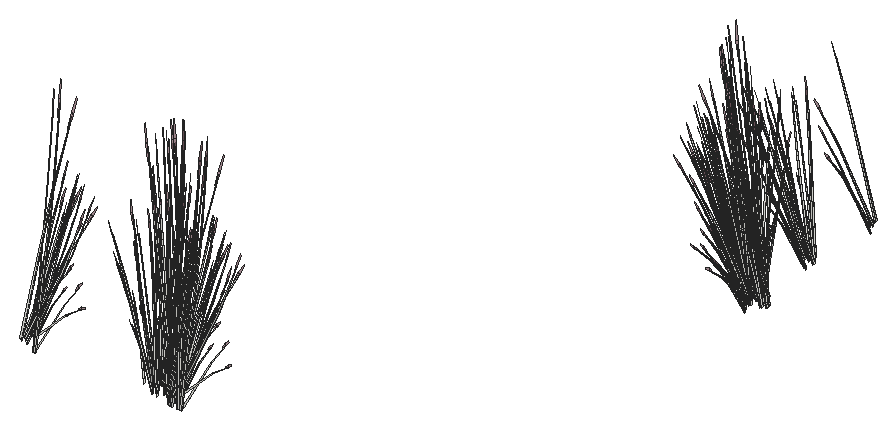
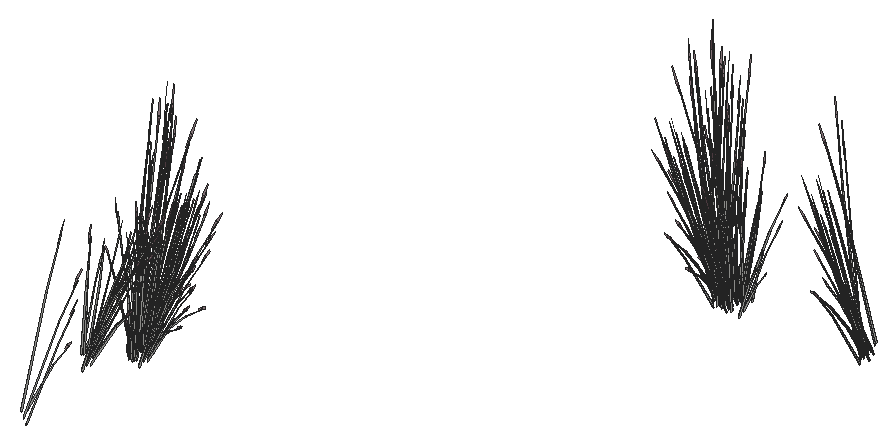
# SketchUp Ruby script. Lengths in inches.
U = 1.inch
M = Sketchup.active_model
def pt(a) = Geom::Point3d.new(a.map { |v| v * U })
def face(e, loops, mat)
  f = e.add_face(loops[0].map { |a| pt(a) })
  loops[1..].each { |l| e.add_face(l.map { |a| pt(a) }).erase! }
  f.material = f.back_material = mat if mat
  f
end
# faces: each face lists its corners as indices into pts; further lists are holes
def faces(e, pts, list, mat = nil) = list.each { |f| face(e, (f[0].is_a?(Array) ? f : [f]).map { |l| l.map { |i| pts[i] } }, mat) }
# xy, xz, yz: faces in a plane at the given z, y or x. An outline is a flat list of corners, or four numbers for a rectangle; further outlines are holes
def ring(l) = l.size == 4 ? [[l[0], l[1]], [l[2], l[1]], [l[2], l[3]], [l[0], l[3]]] : l.each_slice(2).to_a
def flat(e, list, mat, &to3) = list.each { |f| face(e, (f[0].is_a?(Array) ? f : [f]).map { |l| ring(l).map { |u, v| to3.(u, v) } }, mat) }
def xy(e, z, list, mat = nil) = flat(e, list, mat) { |x, y| [x, y, z] }
def xz(e, y, list, mat = nil) = flat(e, list, mat) { |x, z| [x, y, z] }
def yz(e, x, list, mat = nil) = flat(e, list, mat) { |y, z| [x, y, z] }
def lines(e, pts, list) = list.each { |a, b| e.add_line(pt(pts[a]), pt(pts[b])) }
# prism: a flat outline (further loops are holes) pulled along v
def prism(e, loops, v, mat = nil)
  f = face(e, loops, mat); d = Geom::Vector3d.new(v.map { |x| x * U })
  f.pushpull(f.normal.samedirection?(d) ? d.length : -d.length)
end
def box(e, o, s, mat = nil) = prism(e, [[o, [o[0] + s[0], o[1], o[2]], [o[0] + s[0], o[1] + s[1], o[2]], [o[0], o[1] + s[1], o[2]]]], [0, 0, s[2]], mat)
def at(x, y, z, deg = 0) = Geom::Transformation.translation(pt([x, y, z])) * Geom::Transformation.rotation(ORIGIN, Z_AXIS, deg.degrees)
def axes(o, x, y, z) = Geom::Transformation.new([*x, 0, *y, 0, *z, 0, *pt(o).to_a, 1])
def part(name) = M.definitions.add(name)
# library, detail: a bought-in or finely detailed component or shape, given as its bounding box
def library(name, o, s) = part(name).tap { |d| box(d.entities, o, s) }
def detail(e, o, s) = box(e.add_group.entities, o, s)
def put(e, d, t, mat = nil) = e.add_instance(d, t).tap { |i| i.material = mat if mat }
def group(e, t, mat = nil) = e.add_group.tap { |g| g.transformation = t; g.material = mat if mat }.entities
root = M.entities
M.materials.add("LightPink_Translucent").color = [144, 107, 117]
M.materials["LightPink_Translucent"].alpha = 0.75
c1 = part("blade")
p = [[2.15,0.21,22],[0,0.17,0],[0.09,0.45,0],[2.18,0.31,22],[2.29,0.31,22],[0.38,0.45,0],
  [2.48,0.24,33],[2.49,0.24,33],[2.48,0.22,33]]
faces(c1.entities,p,[[0,1,2,3],[4,5,2,3],[6,3,4,7],[8,0,3,6]])
c2 = part("seeds")
p = [[0.3,-0.1,1.38],[-0.01,-0.03,1.59],[-0.01,-0.03,0.03],[0.14,-0.07,-0.07],[0.29,-0.03,3],[0.15,0.01,3.11]]
faces(c2.entities,p,[[0,1,2,3],[1,0,4,5]],"LightPink_Translucent")
c3 = part("blade with seeds")
put(c3.entities,c1,at(0,0,0))
put(c3.entities,c2,axes([2.4,0.25,30.99],[1.5799,-0.05474,1.17369],[-0.12525,1.92788,0.29478],[-0.07173,-0.02425,1.56792]))
put(root,c3,axes([421.09,14.8,-3.8],[0.76598,0.27433,0],[-0.36864,0.57001,0],[0,0,1.74954]))
put(root,c3,axes([386.9,14.48,-1.28],[0.16299,-0.01033,1.74944],[0.44707,-0.47471,-0.27667],[0.28992,0.06266,0.14031]))
put(root,c3,axes([423.32,14.48,-1.28],[0.16299,-0.01033,1.74944],[0.44707,-0.47471,-0.27667],[0.28992,0.06266,0.14031]))
put(root,c3,axes([421.4,15.4,-3.81],[-0.46912,-0.61443,-0.05142],[0.79476,-0.34146,0.51607],[-0.19584,0.0585,1.6363]))
put(root,c3,axes([421.23,13.92,-3.38],[0.56134,0.36712,0.1448],[-0.46823,0.41419,-0.41347],[-0.13033,0.05599,1.26744]))
put(root,c3,axes([416.8,14.01,-1.27],[-0.18844,-0.56237,0.48003],[0.73919,-0.0976,0.3958],[-0.21785,0.13226,0.9933]))
put(root,c3,axes([416.65,13.9,-1.27],[-0.52161,-0.25698,0.0643],[0.30368,-0.36595,0.50621],[-0.16723,0.11831,0.77189]))
put(root,c3,axes([416.89,13.23,-2.125],[0.26363,-0.12925,1.71376],[0.22195,0.59723,0.13857],[-0.41388,0.13498,0.73262]))
put(root,c3,axes([386.27,14.55,-1.02],[0.75952,0.01471,-0.71045],[-0.05101,0.61953,0.08574],[0.32177,0.06538,1.00501]))
put(root,c3,axes([422.6875,14.55,-1.02],[0.75952,0.01471,-0.71045],[-0.05101,0.61953,0.08574],[0.32177,0.06538,1.00501]))
put(root,c3,axes([421.83,15.05,-3.52],[0.7111,-0.30552,0.49651],[0.42504,0.54784,0],[-0.16196,0.06958,1.57504]))
put(root,c3,axes([420.82,14.57,-3.71],[0.33034,0.70197,-0.06012],[-0.94388,0.24598,0],[0.01154,0.02451,1.72173]))
put(root,c3,axes([421.19,15.32,-3.97],[-0.70886,-0.15119,-0.30978],[0.17848,-0.53243,0.30978],[-0.1429,0.0614,1.38974]))
put(root,c3,axes([416.07,14.24,-3.41],[0.26405,0.05016,1.43002],[0.17019,0.51235,-0.30754],[-0.35868,0.0959,0.61141]))
put(root,c3,axes([417.25,13.83,-0.95],[0.66138,-0.08733,0.35414],[0.17464,0.49921,-0.4572],[-0.18953,0.13408,0.87481]))
put(root,c3,axes([387.51,13.29,-3.625],[0.95008,0,0],[0,0.68292,-0.51607],[0,0.15554,1.63711]))
put(root,c3,axes([423.93,13.29,-3.625],[0.95008,0,0],[0,0.68292,-0.51607],[0,0.15554,1.63711]))
put(root,c3,axes([414.71,13.6,-1.29],[0.09697,0.01639,1.77383],[0.29997,0.53988,-0.16761],[-0.1985,0.1417,0.31391]))
put(root,c3,axes([423.55,13.64,-3.8],[-0.94962,-0.00489,-0.04976],[0,-0.68292,0.49943],[-0.02984,0.15546,1.58352]))
put(root,c3,axes([421.49,13.05,-3.33],[0.85568,0.29155,-0.29095],[-0.41201,0.61537,-0.50002],[0.02689,0.15109,1.59708]))
put(root,c3,axes([415.52,15.32,-3.23],[0.31665,-0.27694,1.1486],[0.12495,0.43841,0.84392],[-0.22883,0.0785,0.25299]))
put(root,c3,axes([386.72,14.81,-1.47],[0.43232,0.38257,-0.35414],[-0.49364,0.36215,0.4572],[0.25081,0.0551,0.87481]))
put(root,c3,axes([423.14,14.81,-1.47],[0.43232,0.38257,-0.35414],[-0.49364,0.36215,0.4572],[0.25081,0.0551,0.87481]))
put(root,c3,axes([423.35,13.74,-3.97],[-0.53038,0.38124,-0.30978],[-0.53038,-0.38124,0.30978],[0,0.1228,1.38974]))
put(root,c3,axes([421.0625,13.78,-3.33],[0.08854,0.69723,-0.29095],[-0.92215,0.04216,-0.50002],[-0.16238,0.09287,1.59708]))
put(root,c3,axes([386.5,14.95,-1.27],[-0.03826,0.46465,0.0643],[-0.57772,-0.01274,0.50621],[0.2213,0.04862,0.77189]))
put(root,c3,axes([422.92,14.95,-1.27],[-0.03826,0.46465,0.0643],[-0.57772,-0.01274,0.50621],[0.2213,0.04862,0.77189]))
put(root,c3,axes([421.4,13.51,-3.79],[-0.36864,0.55059,-0.44739],[-0.76598,-0.26498,0.21531],[0,0.12692,1.43643]))
put(root,c3,axes([416.71,14.12,-1.47],[-0.66138,0.08733,-0.35414],[-0.17464,-0.49921,0.4572],[-0.18953,0.13408,0.87481]))
put(root,c3,axes([386.56,14.81,-1.27],[-0.56024,0.40262,0.48003],[-0.48318,-0.42758,0.3958],[0.26285,0.07427,0.9933]))
put(root,c3,axes([422.97,14.81,-1.27],[-0.56024,0.40262,0.48003],[-0.48318,-0.42758,0.3958],[0.26285,0.07427,0.9933]))
put(root,c3,axes([415.75,15.24,-0.35],[0.67048,0.16311,-0.06488],[-0.20625,0.50201,-0.29416],[-0.10966,0.07622,0.97024]))
put(root,c3,axes([420.51,14.3125,-3.94],[-0.51177,0.45928,-0.62353],[-0.63575,-0.41646,-0.16365],[-0.20507,0.11457,1.37633]))
put(root,c3,axes([384.77,15.27,-0.95],[-0.11735,-0.49217,0.35414],[0.67083,-0.12996,-0.4572],[0.18018,0.14104,0.87481]))
put(root,c3,axes([421.19,15.27,-0.95],[-0.11735,-0.49217,0.35414],[0.67083,-0.12996,-0.4572],[0.18018,0.14104,0.87481]))
put(root,c3,axes([421.42,15.09,-3.67],[0.95122,0.19861,0.30756],[-0.23797,0.7099,-0.36492],[-0.15744,0.08885,1.64885]))
put(root,c3,axes([421.35,15.57,-3.98],[-0.7111,0.30552,-0.49651],[-0.42504,-0.54784,0],[-0.16196,0.06958,1.57504]))
put(root,c3,axes([387.3,13.76,-3.98],[0,0.61104,-0.49651],[-0.85008,0,0],[0,0.13917,1.57504]))
put(root,c3,axes([423.71,13.76,-3.98],[0,0.61104,-0.49651],[-0.85008,0,0],[0,0.13917,1.57504]))
put(root,c3,axes([385.17,13.83,-2.125],[-0.28223,-0.10528,1.71376],[0.58406,-0.44165,0.13857],[0.36402,0.19924,0.73262]))
put(root,c3,axes([421.59,13.83,-2.125],[-0.28223,-0.10528,1.71376],[0.58406,-0.44165,0.13857],[0.36402,0.19924,0.73262]))
put(root,c3,axes([385.23,12.44,-1.53],[-0.65655,-0.31748,1.38283],[0.69326,-0.49431,0.59665],[0.21183,0.29789,1.33663]))
put(root,c3,axes([421.64,12.44,-1.53],[-0.65655,-0.31748,1.38283],[0.69326,-0.49431,0.59665],[0.21183,0.29789,1.33663]))
put(root,c3,axes([416.91,13.78,-0.97],[0.70283,0.33692,-0.1216],[-0.40491,0.48793,-0.67495],[-0.19857,0.16961,1.02557]))
put(root,c3,axes([386.22,15.02,-3.23],[-0.4278,-0.1757,1.1486],[0.5524,-0.17852,0.84392],[0.14899,0.15122,0.25299]))
put(root,c3,axes([422.63,15.02,-3.23],[-0.4278,-0.1757,1.1486],[0.5524,-0.17852,0.84392],[0.14899,0.15122,0.25299]))
put(root,c3,axes([384.71,15.53,-0.97],[0.45276,-0.52302,-0.1216],[0.65568,0.30132,-0.67495],[0.22792,0.14777,1.02557]))
put(root,c3,axes([421.13,15.53,-0.97],[0.45276,-0.52302,-0.1216],[0.65568,0.30132,-0.67495],[0.22792,0.14777,1.02557]))
put(root,c3,axes([417.86,13.63,-2.125],[0.18977,-0.18775,1.71376],[0.47917,0.50677,0.13857],[-0.32866,0.23079,0.73262]))
put(root,c3,axes([417.26,14.18,-1.32],[0.19519,0.55794,-0.51099],[-0.73919,0.0976,-0.3958],[-0.21183,0.14986,0.97773]))
put(root,c3,axes([418.15,14.82,-0.95],[0.5141,-0.32171,0.35414],[0.48666,0.36734,-0.4572],[-0.07405,0.18664,0.87481]))
put(root,c3,axes([422,15.47,-3.625],[0.47504,0.61229,0],[-0.79476,0.34146,-0.51607],[-0.18101,0.07777,1.63711]))
put(root,c3,axes([384.12,15.96,-1.29],[0.00225,-0.07398,1.77383],[0.65113,-0.32638,-0.16761],[0.22617,0.1165,0.31391]))
put(root,c3,axes([420.54,15.96,-1.29],[0.00225,-0.07398,1.77383],[0.65113,-0.32638,-0.16761],[0.22617,0.1165,0.31391]))
put(root,c3,axes([386.34,15.68,-4.51],[0.05536,-0.08822,1.76342],[0.69692,-0.25981,-0.26939],[0.21129,0.13447,0.30037]))
put(root,c3,axes([422.75,15.68,-4.51],[0.05536,-0.08822,1.76342],[0.69692,-0.25981,-0.26939],[0.21129,0.13447,0.30037]))
put(root,c3,axes([421.59,13.05,-3.16],[-0.02076,-0.57531,1.41272],[0.93937,0.14913,0.59816],[-0.22217,0.31481,1.3335]))
put(root,c3,axes([421.83,13.67,-3.91],[0.2786,0.55945,-0.69212],[-0.80253,0.20149,-0.18165],[0.03079,0.18945,1.52773]))
put(root,c3,axes([417.68,15.11,-1.27],[-0.62439,-0.02847,0.0643],[0.01712,-0.42991,0.50621],[-0.06534,0.16468,0.77189]))
put(root,c3,axes([416.35,15.6,-4.51],[0.10192,0.06105,1.76342],[0.17281,0.56562,-0.26939],[-0.22588,0.12062,0.30037]))
put(root,c3,axes([417.88,15.15,-1.27],[-0.54105,-0.41691,0.48003],[0.57458,-0.35956,0.3958],[-0.0998,0.1956,0.9933]))
put(root,c3,axes([385.25,15.27,-1.32],[0.74975,-0.14525,-0.51099],[0.13115,0.55007,-0.3958],[0.20138,0.15763,0.97773]))
put(root,c3,axes([421.67,15.27,-1.32],[0.74975,-0.14525,-0.51099],[0.13115,0.55007,-0.3958],[0.20138,0.15763,0.97773]))
put(root,c3,axes([419.59,15.35,-0.95],[0.22906,-0.4699,0.35414],[0.66828,0.13705,-0.4572],[0.06128,0.18919,0.87481]))
put(root,c3,axes([386.28,15.82,-3.33],[-0.48723,-0.01916,1.0506],[0.32177,-0.40701,0.58006],[0.19248,0.1446,0.8241]))
put(root,c3,axes([422.7,15.82,-3.33],[-0.48723,-0.01916,1.0506],[0.32177,-0.40701,0.58006],[0.19248,0.1446,0.8241]))
put(root,c3,axes([384.88,15.72,-1.27],[-0.34533,0.38816,0.0643],[-0.49176,-0.22599,0.50621],[0.15898,0.12445,0.77189]))
put(root,c3,axes([421.3,15.72,-1.27],[-0.34533,0.38816,0.0643],[-0.49176,-0.22599,0.50621],[0.15898,0.12445,0.77189]))
put(root,c3,axes([420.49,17.03,-0.35],[0.52505,-0.35054,-0.06488],[0.48109,0.38392,-0.29416],[0.03387,0.10878,0.97024]))
put(root,c3,axes([385.03,15.61,-1.27],[-0.75571,0.14023,0.48003],[-0.13115,-0.55007,0.3958],[0.17773,0.16212,0.9933]))
put(root,c3,axes([421.44,15.61,-1.27],[-0.75571,0.14023,0.48003],[-0.13115,-0.55007,0.3958],[0.17773,0.16212,0.9933]))
put(root,c3,axes([417.71,14.09,-2.125],[0.14147,-0.21002,1.71376],[0.59349,0.43464,0.13857],[-0.26773,0.27089,0.73262]))
put(root,c3,axes([384.69,14.84,-3.41],[0.01341,-0.20255,1.43002],[0.64074,-0.22625,-0.30754],[0.1978,0.24243,0.61141]))
put(root,c3,axes([421.11,14.84,-3.41],[0.01341,-0.20255,1.43002],[0.64074,-0.22625,-0.30754],[0.1978,0.24243,0.61141]))
put(root,c3,axes([419.38,15.77,-1.27],[-0.55987,0.20767,0.0643],[-0.27403,-0.37869,0.50621],[0.05407,0.16693,0.77189]))
put(root,c3,axes([417.88,15.28,-1.47],[-0.5141,0.32171,-0.35414],[-0.48666,-0.36734,0.4572],[-0.07405,0.18664,0.87481]))
put(root,c3,axes([416.11,15.18,-1.28],[-0.01889,0.12092,1.74944],[0.53598,0.42065,-0.27667],[-0.14032,0.19892,0.14031]))
put(root,c3,axes([417.82,14.91,-0.6],[0.83505,0.03027,-0.13498],[-0.02282,0.57322,-0.74919],[-0.05801,0.22077,1.13838]))
put(root,c3,axes([419.36,15.55,-0.97],[0.74352,-0.28449,-0.1216],[0.36538,0.50492,-0.67495],[0.0981,0.21277,1.02557]))
put(root,c3,axes([419.58,15.73,-0.9375],[-0.74868,-0.15974,0.53283],[0.25601,-0.52518,0.43934],[0.04499,0.20653,1.10256]))
put(root,c3,axes([418.21,16.53,-3.23],[-0.01966,-0.36332,1.1486],[0.49135,0.25914,0.84392],[-0.09663,0.17317,0.25299]))
put(root,c3,axes([419.5,15.66,-4.51],[0.12297,-0.03325,1.76342],[0.73967,0.18301,-0.26939],[0.02163,0.20626,0.30037]))
put(root,c3,axes([418.39,15.125,-1],[0.54391,0.41056,-0.5672],[-0.57458,0.35956,-0.43934],[-0.08276,0.2086,1.08528]))
put(root,c3,axes([417.8,15.74,-3.18],[0.69024,-0.1082,0.06507],[0.15868,0.43593,-0.86304],[-0.04376,0.22067,0.7736]))
put(root,c3,axes([420,15.52,-1.32],[0.7469,0.15318,-0.51099],[-0.25601,0.52518,-0.3958],[0.06849,0.21144,0.97773]))
put(root,c3,axes([384.01,14.4375,-2.125],[-0.17368,-0.19618,1.71376],[0.80256,-0.16516,0.13857],[0.18139,0.30799,0.73262]))
put(root,c3,axes([420.43,14.4375,-2.125],[-0.17368,-0.19618,1.71376],[0.80256,-0.16516,0.13857],[0.18139,0.30799,0.73262]))
put(root,c3,axes([419.66,15.84,-1.47],[-0.22906,0.4699,-0.35414],[-0.66828,-0.13705,0.4572],[0.06128,0.18919,0.87481]))
put(root,c3,axes([418.22,14.9375,-0.66],[-0.01977,0.56521,-0.7886],[-0.83252,-0.03796,0.09517],[-0.08786,0.23945,1.11556]))
put(root,c3,axes([416.05,16.42,-1.29],[0.0862,-0.03689,1.77383],[0.71245,0.24539,-0.16761],[-0.01674,0.20431,0.31391]))
put(root,c3,axes([419.01,14.54,-2.125],[-0.0186,-0.23452,1.71376],[0.80601,0.15558,0.13857],[-0.04985,0.33422,0.73262]))
put(root,c3,axes([419.73,15.42,-1.02],[0.36264,0.49684,-0.71045],[-0.74649,0.27689,0.08574],[0.0848,0.24006,1.00501]))
put(root,c3,axes([417.63,16.2,-3.41],[0.23977,-0.09639,1.43002],[0.59198,0.29065,-0.30754],[-0.1762,0.25149,0.61141]))
put(root,c3,axes([419.1875,16.68,-1.28],[0.09631,0.0984,1.74944],[0.77725,0.03866,-0.27667],[0.07816,0.217,0.14031]))
put(root,c3,axes([417.94,15.73,-2.64],[0.01669,-0.31544,1.54345],[0.75083,0.16661,0.21329],[-0.06506,0.33618,0.72882]))
put(root,c3,axes([491.26,105.73,3.07],[0.17368,0.19618,1.71376],[-0.80256,0.16516,0.13857],[-0.18139,-0.30799,0.73262]))
put(root,c3,axes([492.59,104.43,3.91],[-0.11621,-0.08567,1.74944],[-0.77555,0.05431,-0.27667],[-0.12378,-0.20491,0.14031]))
put(root,c3,axes([491.04,105.21,1.78],[-0.04601,0.19989,1.43002],[-0.67263,0.16733,-0.30754],[-0.15723,-0.25836,0.61141]))
put(root,c3,axes([491.79,104.15,3.9],[-0.01417,0.07324,1.77383],[-0.6991,0.2658,-0.16761],[-0.20573,-0.13587,0.31391]))
put(root,c3,axes([491.64,105.45,4.29],[0.84639,-0.15705,0.53763],[0.14689,0.61608,0.4433],[-0.19906,-0.18157,1.11249]))
put(root,c3,axes([490.8125,104.89,1.96],[0.39634,0.21267,1.1486],[-0.57721,0.12784,0.84392],[-0.1235,-0.16344,0.25299]))
put(root,c3,axes([491.77,106.02,4.17],[-0.64788,-0.29534,-0.71045],[0.46044,-0.51755,0.08574],[-0.23473,-0.17635,1.00501]))
put(root,c3,axes([491.54,105.63,3.72],[-0.11735,-0.49217,-0.35414],[0.67083,-0.12996,0.4572],[-0.18018,-0.14104,0.87481]))
put(root,c3,axes([491.83,105.58,3.92],[0.34533,-0.38816,0.0643],[0.49176,0.22599,0.50621],[-0.15898,-0.12445,0.77189]))
put(root,c3,axes([490.5,105.53,0.6875],[-0.0736,0.08049,1.76342],[-0.74378,0.17355,-0.26939],[-0.17968,-0.15788,0.30037]))
put(root,c3,axes([490.1,106.34,3.07],[0.28223,0.10528,1.71376],[-0.58406,0.44165,0.13857],[-0.36402,-0.19924,0.73262]))
put(root,c3,axes([491.47,106.03,3.875],[-0.74975,0.14525,-0.51099],[-0.13115,-0.55007,-0.3958],[-0.20138,-0.15763,0.97773]))
put(root,c3,axes([491.99,105.54,4.62],[-0.50709,0.58578,-0.13619],[-0.73436,-0.33748,-0.75594],[-0.25527,-0.1655,1.14864]))
put(root,c3,axes([490.05,105.375,3.91],[-0.16348,-0.00431,1.74944],[-0.52047,0.43131,-0.27667],[-0.2777,-0.08813,0.14031]))
put(root,c3,axes([493.32,109.36,2.52],[0.65659,0.2464,1.51261],[-0.64324,0.53082,0.59816],[-0.28812,-0.31461,1.26806]))
put(root,c3,axes([491.94,106.03,4.24],[0.11735,0.49217,0.35414],[-0.67083,0.12996,-0.4572],[-0.18018,-0.14104,0.87481]))
put(root,c3,axes([489.93,106.35,4.29],[0.62747,-0.45094,0.53763],[0.54116,0.47889,0.4433],[-0.29439,-0.08318,1.11249]))
put(root,c3,axes([490.21,106.35,3.92],[0.03826,-0.46465,0.0643],[0.57772,0.01274,0.50621],[-0.2213,-0.04862,0.77189]))
put(root,c3,axes([489.99,106.49,3.72],[-0.43232,-0.38257,-0.35414],[0.49364,-0.36215,0.4572],[-0.25081,-0.0551,0.87481]))
put(root,c3,axes([490.04,105.84,1.32],[-0.21918,0.49894,-0.03893],[-0.6746,-0.15348,-0.17649],[-0.10242,-0.08161,0.58215]))
put(root,c3,axes([489.67,108.12,1.57],[-0.95008,0,0],[0,-0.68292,-0.51607],[0,-0.15554,1.63711]))
put(root,c3,axes([489.84,106.9,1.78],[0.14835,0.17012,1.43002],[-0.34183,0.46242,-0.30754],[-0.351,-0.11053,0.61141]))
put(root,c3,axes([490.45,106.75,4.17],[-0.75952,-0.01471,-0.71045],[0.05101,-0.61953,0.08574],[-0.32177,-0.06538,1.00501]))
put(root,c3,axes([490.41,107.94,1.52],[-0.70674,0.51372,0.30756],[-0.70717,-0.50832,-0.36492],[-0.02468,-0.14589,1.64885]))
put(root,c3,axes([489.42,105.74,3.9],[0.05633,0.06098,1.77383],[-0.27155,0.54815,-0.16761],[-0.27501,0.00397,0.31391]))
put(root,c3,axes([492.32,109.01,1.63],[0.20138,-0.72405,-0.23429],[0.95485,0.12621,0.51271],[-0.16685,-0.09999,1.5644]))
put(root,c3,axes([490.2,106.875,3.875],[-0.55171,0.40476,-0.51099],[-0.48318,-0.42758,-0.3958],[-0.28031,-0.06159,0.97773]))
put(root,c3,axes([490.6,106.69,4.24],[0.43232,0.38257,0.35414],[-0.49364,0.36215,-0.4572],[-0.25081,-0.0551,0.87481]))
put(root,c3,axes([488.95,107.41,1.96],[0.48508,-0.04372,1.1486],[-0.3077,0.38525,0.84392],[-0.23971,-0.05779,0.25299]))
put(root,c3,axes([490.49,106.45,4.23],[-0.04068,0.62141,-0.1216],[-0.77029,-0.01698,-0.67495],[-0.29667,-0.04317,1.02557]))
put(root,c3,axes([489.51,107.31,3.07],[0.31515,-0.01384,1.71376],[-0.20907,0.5998,0.13857],[-0.44912,-0.0371,0.73262]))
put(root,c3,axes([492.26,108.72,1.4],[-0.45644,-0.51287,-0.44739],[0.69137,-0.36116,0.21531],[-0.14771,-0.06346,1.43643]))
put(root,c3,axes([491.85,108.91,1.25],[-0.79037,-0.10018,-0.62353],[0.16679,-0.61794,-0.16365],[-0.23587,-0.07488,1.37633]))
put(root,c3,axes([489.375,107.76,3.93],[0.21466,-0.55714,0.48003],[0.70573,0.19051,0.3958],[-0.27753,0.03348,0.9933]))
put(root,c3,axes([489.32,107.61,3.92],[-0.27906,-0.41663,0.0643],[0.50888,-0.20393,0.50621],[-0.22432,0.04024,0.77189]))
put(root,c3,axes([489.31,108.04,0.6875],[0.01927,0.0963,1.76342],[-0.38846,0.5029,-0.26939],[-0.27592,-0.02535,0.30037]))
put(root,c3,axes([491.01,109.85,1.22],[-0.17848,-0.53243,-0.30978],[0.70886,-0.15119,0.30978],[-0.1429,-0.0614,1.38974]))
put(root,c3,axes([490.81,110.08,1.21],[-0.7111,-0.30552,-0.49651],[0.42504,-0.54784,0],[-0.16196,-0.06958,1.57504]))
put(root,c3,axes([489.23,107.82,3.72],[-0.63144,-0.17046,-0.35414],[0.18417,-0.49731,0.4572],[-0.25423,0.0456,0.87481]))
put(root,c3,axes([492.74,109,1.86],[-0.76714,0.40567,-0.29095],[-0.51013,-0.57321,-0.50002],[-0.18927,-0.05821,1.59708]))
put(root,c3,axes([492.67,109.18,1.81],[-0.14658,0.54532,0.1448],[-0.71613,-0.09466,-0.41347],[-0.13033,-0.05599,1.26744]))
put(root,c3,axes([489.89,107.77,4.24],[0.63144,0.17046,0.35414],[-0.18417,0.49731,-0.4572],[-0.25423,0.0456,0.87481]))
put(root,c3,axes([491.15,107.74,2.53],[0.21597,-0.08839,1.77064],[0.07448,0.61717,0.13857],[-0.4678,0.08189,0.63284]))
put(root,c3,axes([493.61,109.1875,1.66],[-0.74193,-0.49181,-0.25192],[0.6243,-0.55226,0.5513],[-0.19979,0.05753,1.68216]))
put(root,c3,axes([491.65,110.13,1.67],[0.7111,0.30552,0.49651],[-0.42504,0.54784,0],[-0.16196,-0.06958,1.57504]))
put(root,c3,axes([488.83,108.15,3.91],[-0.12407,0.07933,1.74944],[0.01055,0.57963,-0.27667],[-0.2844,0.07538,0.14031]))
put(root,c3,axes([489.66,108.07,3.875],[-0.20584,0.55581,-0.51099],[-0.70573,-0.19051,-0.3958],[-0.28414,0.05097,0.97773]))
put(root,c3,axes([489.625,107.6,4.23],[0.38229,0.5533,-0.1216],[-0.6785,0.2719,-0.67495],[-0.28593,0.073,1.02557]))
put(root,c3,axes([491.24,110.45,1.57],[-0.47504,0.61229,0],[-0.79476,-0.34146,-0.51607],[-0.18101,-0.07777,1.63711]))
put(root,c3,axes([493.23,109.08,1.4],[-0.82508,0.03772,-0.44739],[-0.07462,-0.62614,0.21531],[-0.14771,0.06346,1.43643]))
put(root,c3,axes([489.54,109.15,3.93],[-0.18844,-0.56237,0.48003],[0.73919,-0.0976,0.3958],[-0.21785,0.13226,0.9933]))
put(root,c3,axes([489.4,109.04,3.92],[-0.52161,-0.25698,0.0643],[0.30368,-0.36595,0.50621],[-0.16723,0.11831,0.77189]))
put(root,c3,axes([489.64,108.36,3.07],[0.26363,-0.12925,1.71376],[0.22195,0.59723,0.13857],[-0.41388,0.13498,0.73262]))
put(root,c3,axes([488.82,109.38,1.78],[0.26405,0.05016,1.43002],[0.17019,0.51235,-0.30754],[-0.35868,0.0959,0.61141]))
put(root,c3,axes([490,108.96,4.24],[0.66138,-0.08733,0.35414],[0.17464,0.49921,-0.4572],[-0.18953,0.13408,0.87481]))
put(root,c3,axes([487.45,108.74,3.9],[0.09697,0.01639,1.77383],[0.29997,0.53988,-0.16761],[-0.1985,0.1417,0.31391]))
put(root,c3,axes([488.26,110.45,1.96],[0.31665,-0.27694,1.1486],[0.12495,0.43841,0.84392],[-0.22883,0.0785,0.25299]))
put(root,c3,axes([489.46,109.26,3.72],[-0.66138,0.08733,-0.35414],[-0.17464,-0.49921,0.4572],[-0.18953,0.13408,0.87481]))
put(root,c3,axes([488.5,110.38,4.84],[0.67048,0.16311,-0.06488],[-0.20625,0.50201,-0.29416],[-0.10966,0.07622,0.97024]))
put(root,c3,axes([493.25,109.45,1.25],[-0.51177,0.45928,-0.62353],[-0.63575,-0.41646,-0.16365],[-0.20507,0.11457,1.37633]))
put(root,c3,axes([489.66,108.91,4.23],[0.70283,0.33692,-0.1216],[-0.40491,0.48793,-0.67495],[-0.19857,0.16961,1.02557]))
put(root,c3,axes([490.6,108.76,3.07],[0.18977,-0.18775,1.71376],[0.47917,0.50677,0.13857],[-0.32866,0.23079,0.73262]))
put(root,c3,axes([490,109.3125,3.875],[0.19519,0.55794,-0.51099],[-0.73919,0.0976,-0.3958],[-0.21183,0.14986,0.97773]))
put(root,c3,axes([490.43,110.25,3.92],[-0.62439,-0.02847,0.0643],[0.01712,-0.42991,0.50621],[-0.06534,0.16468,0.77189]))
put(root,c3,axes([489.1,110.74,0.6875],[0.10192,0.06105,1.76342],[0.17281,0.56562,-0.26939],[-0.22588,0.12062,0.30037]))
put(root,c3,axes([490.625,110.29,3.93],[-0.54105,-0.41691,0.48003],[0.57458,-0.35956,0.3958],[-0.0998,0.1956,0.9933]))
put(root,c3,axes([490.46,109.23,3.07],[0.14147,-0.21002,1.71376],[0.59349,0.43464,0.13857],[-0.26773,0.27089,0.73262]))
put(root,c3,axes([490.62,110.41,3.72],[-0.5141,0.32171,-0.35414],[-0.48666,-0.36734,0.4572],[-0.07405,0.18664,0.87481]))
put(root,c3,axes([488.85,110.32,3.91],[-0.01889,0.12092,1.74944],[0.53598,0.42065,-0.27667],[-0.14032,0.19892,0.14031]))
put(root,c3,axes([490.95,111.66,1.96],[-0.01966,-0.36332,1.1486],[0.49135,0.25914,0.84392],[-0.09663,0.17317,0.25299]))
put(root,c3,axes([490.97,110.07,4.53],[-0.01977,0.56521,-0.7886],[-0.83252,-0.03796,0.09517],[-0.08786,0.23945,1.11556]))
put(root,c3,axes([488.79,111.56,3.9],[0.0862,-0.03689,1.77383],[0.71245,0.24539,-0.16761],[-0.01674,0.20431,0.31391]))
put(root,c3,axes([490.375,111.34,1.78],[0.23977,-0.09639,1.43002],[0.59198,0.29065,-0.30754],[-0.1762,0.25149,0.61141]))
put(root,c3,axes([493.73,119.48,6.68],[0.28223,0.10528,1.71376],[-0.58406,0.44165,0.13857],[-0.36402,-0.19924,0.73262]))
put(root,c3,axes([490.6875,110.87,2.56],[0.01669,-0.31544,1.54345],[0.75083,0.16661,0.21329],[-0.06506,0.33618,0.72882]))
put(root,c3,axes([493.62,119.63,7.33],[-0.43232,-0.38257,-0.35414],[0.49364,-0.36215,0.4572],[-0.25081,-0.0551,0.87481]))
put(root,c3,axes([493.46,120.04,5.39],[0.14835,0.17012,1.43002],[-0.34183,0.46242,-0.30754],[-0.351,-0.11053,0.61141]))
put(root,c3,axes([494.07,119.89,7.78],[-0.75952,-0.01471,-0.71045],[0.05101,-0.61953,0.08574],[-0.32177,-0.06538,1.00501]))
put(root,c3,axes([493.82,120.01,7.48],[-0.55171,0.40476,-0.51099],[-0.48318,-0.42758,-0.3958],[-0.28031,-0.06159,0.97773]))
put(root,c3,axes([492.58,120.55,5.57],[0.48508,-0.04372,1.1486],[-0.3077,0.38525,0.84392],[-0.23971,-0.05779,0.25299]))
put(root,c3,axes([493.13,120.44,6.68],[0.31515,-0.01384,1.71376],[-0.20907,0.5998,0.13857],[-0.44912,-0.0371,0.73262]))
put(root,c3,axes([492.93,121.18,4.29],[0.01927,0.0963,1.76342],[-0.38846,0.5029,-0.26939],[-0.27592,-0.02535,0.30037]))
put(root,c3,axes([492.85,120.96,7.33],[-0.63144,-0.17046,-0.35414],[0.18417,-0.49731,0.4572],[-0.25423,0.0456,0.87481]))
put(root,c3,axes([494.78,120.875,6.14],[0.21597,-0.08839,1.77064],[0.07448,0.61717,0.13857],[-0.4678,0.08189,0.63284]))
put(root,c3,axes([493.29,121.21,7.48],[-0.20584,0.55581,-0.51099],[-0.70573,-0.19051,-0.3958],[-0.28414,0.05097,0.97773]))
put(root,c3,axes([493.26,121.5,6.68],[0.26363,-0.12925,1.71376],[0.22195,0.59723,0.13857],[-0.41388,0.13498,0.73262]))
put(root,c3,axes([492.44,122.52,5.39],[0.26405,0.05016,1.43002],[0.17019,0.51235,-0.30754],[-0.35868,0.0959,0.61141]))
put(root,c3,axes([491.89,123.59,5.57],[0.31665,-0.27694,1.1486],[0.12495,0.43841,0.84392],[-0.22883,0.0785,0.25299]))
put(root,c3,axes([493.09,122.39,7.33],[-0.66138,0.08733,-0.35414],[-0.17464,-0.49921,0.4572],[-0.18953,0.13408,0.87481]))
put(root,c3,axes([494.23,121.9,6.68],[0.18977,-0.18775,1.71376],[0.47917,0.50677,0.13857],[-0.32866,0.23079,0.73262]))
put(root,c3,axes([493.63,122.45,7.48],[0.19519,0.55794,-0.51099],[-0.73919,0.0976,-0.3958],[-0.21183,0.14986,0.97773]))
put(root,c3,axes([492.72,123.875,4.29],[0.10192,0.06105,1.76342],[0.17281,0.56562,-0.26939],[-0.22588,0.12062,0.30037]))
put(root,c3,axes([494.08,122.36,6.68],[0.14147,-0.21002,1.71376],[0.59349,0.43464,0.13857],[-0.26773,0.27089,0.73262]))
put(root,c3,axes([491.34,144.18,3.07],[0.17368,0.19618,1.71376],[-0.80256,0.16516,0.13857],[-0.18139,-0.30799,0.73262]))
put(root,c3,axes([491.12,143.66,1.78],[-0.04601,0.19989,1.43002],[-0.67263,0.16733,-0.30754],[-0.15723,-0.25836,0.61141]))
put(root,c3,axes([491.87,142.6,3.9],[-0.01417,0.07324,1.77383],[-0.6991,0.2658,-0.16761],[-0.20573,-0.13587,0.31391]))
put(root,c3,axes([491.72,143.9,4.29],[0.84639,-0.15705,0.53763],[0.14689,0.61608,0.4433],[-0.19906,-0.18157,1.11249]))
